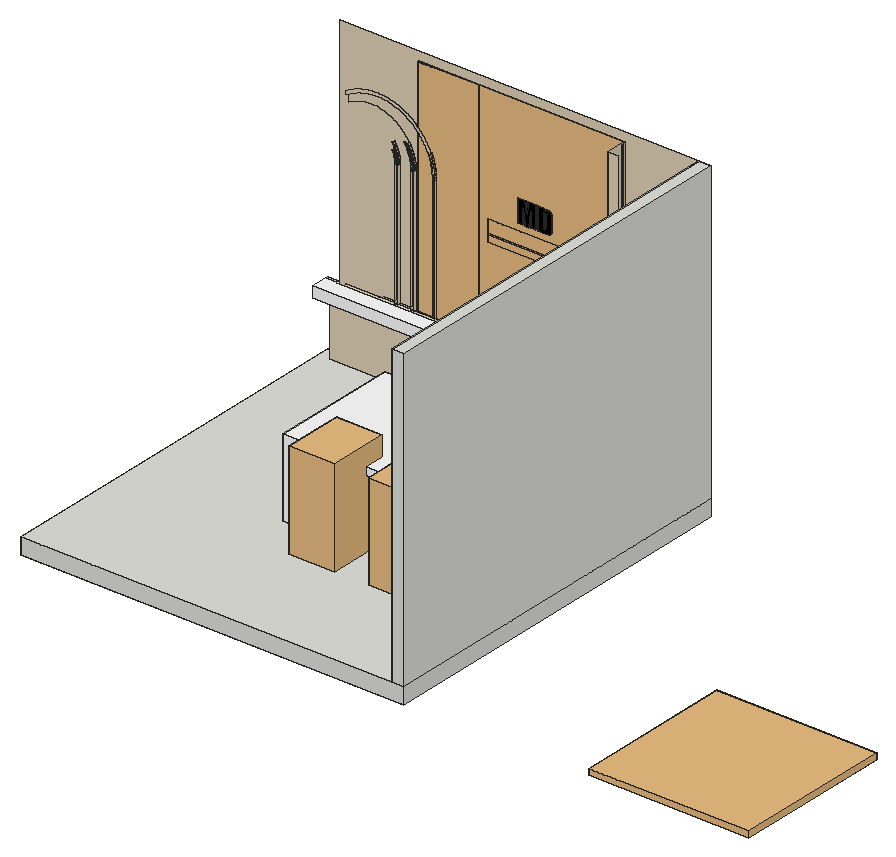
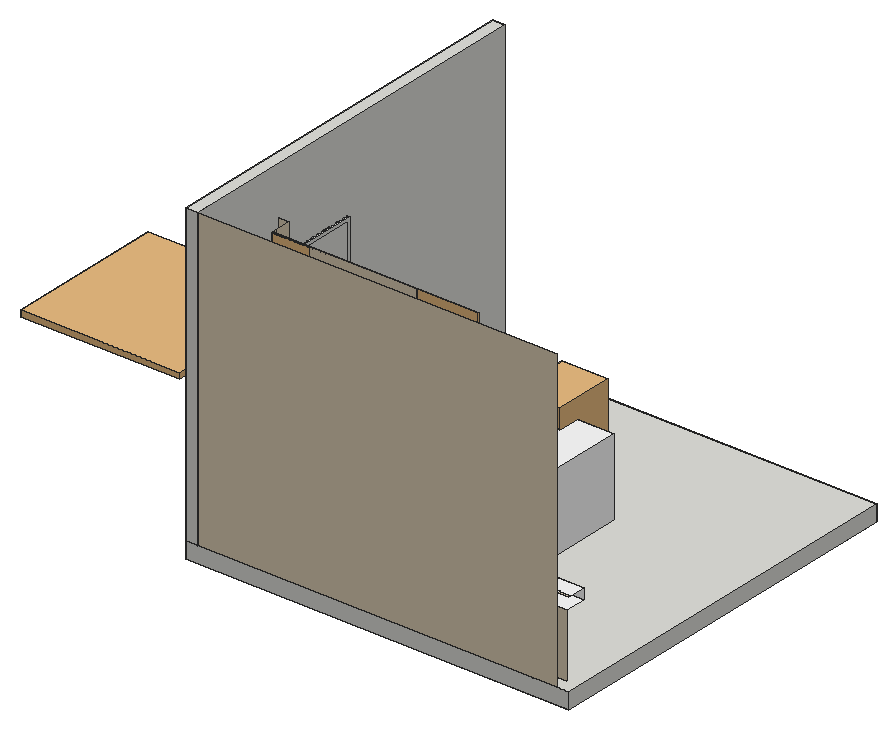
# SketchUp Ruby script. Lengths in inches.
U = 1.inch
M = Sketchup.active_model
def pt(a) = Geom::Point3d.new(a.map { |v| v * U })
def face(e, loops, mat)
  f = e.add_face(loops[0].map { |a| pt(a) })
  loops[1..].each { |l| e.add_face(l.map { |a| pt(a) }).erase! }
  f.material = f.back_material = mat if mat
  f
end
# faces: each face lists its corners as indices into pts; further lists are holes
def faces(e, pts, list, mat = nil) = list.each { |f| face(e, (f[0].is_a?(Array) ? f : [f]).map { |l| l.map { |i| pts[i] } }, mat) }
# xy, xz, yz: faces in a plane at the given z, y or x. An outline is a flat list of corners, or four numbers for a rectangle; further outlines are holes
def ring(l) = l.size == 4 ? [[l[0], l[1]], [l[2], l[1]], [l[2], l[3]], [l[0], l[3]]] : l.each_slice(2).to_a
def flat(e, list, mat, &to3) = list.each { |f| face(e, (f[0].is_a?(Array) ? f : [f]).map { |l| ring(l).map { |u, v| to3.(u, v) } }, mat) }
def xy(e, z, list, mat = nil) = flat(e, list, mat) { |x, y| [x, y, z] }
def xz(e, y, list, mat = nil) = flat(e, list, mat) { |x, z| [x, y, z] }
def yz(e, x, list, mat = nil) = flat(e, list, mat) { |y, z| [x, y, z] }
def lines(e, pts, list) = list.each { |a, b| e.add_line(pt(pts[a]), pt(pts[b])) }
# prism: a flat outline (further loops are holes) pulled along v
def prism(e, loops, v, mat = nil)
  f = face(e, loops, mat); d = Geom::Vector3d.new(v.map { |x| x * U })
  f.pushpull(f.normal.samedirection?(d) ? d.length : -d.length)
end
def box(e, o, s, mat = nil) = prism(e, [[o, [o[0] + s[0], o[1], o[2]], [o[0] + s[0], o[1] + s[1], o[2]], [o[0], o[1] + s[1], o[2]]]], [0, 0, s[2]], mat)
def at(x, y, z, deg = 0) = Geom::Transformation.translation(pt([x, y, z])) * Geom::Transformation.rotation(ORIGIN, Z_AXIS, deg.degrees)
def axes(o, x, y, z) = Geom::Transformation.new([*x, 0, *y, 0, *z, 0, *pt(o).to_a, 1])
def part(name) = M.definitions.add(name)
# library, detail: a bought-in or finely detailed component or shape, given as its bounding box
def library(name, o, s) = part(name).tap { |d| box(d.entities, o, s) }
def detail(e, o, s) = box(e.add_group.entities, o, s)
def put(e, d, t, mat = nil) = e.add_instance(d, t).tap { |i| i.material = mat if mat }
def group(e, t, mat = nil) = e.add_group.tap { |g| g.transformation = t; g.material = mat if mat }.entities
root = M.entities
M.materials.add("Oak Veneered MDF (Z8GPD2)").color = [209, 167, 120]
M.materials.add("Teddy_Brim").color = [225, 210, 185]
M.materials.add("[Color M00]").color = [255, 255, 255]
M.materials.add("[Color M09]").color = [0, 0, 0]
M.materials.add("[Color_000]").color = [255, 255, 255]
M.materials.add("[Color_D05]1").color = [255, 242, 204]
c1 = library("Group10\#1",[-11.375,-42,0],[22.75,84,0.5])
c2 = library("silla generica",[-12.64,0.67,0],[23.23,30.27,48.95])
c3 = part("MD")
prism(c3.entities,[[[3.42,4,0],[3.42,0,0],[2.51,0,0],[2.51,2.7,0],[2.14,0,0],[1.5,0,0],[1.12,2.64,0],[1.12,0,0],[0.21,0,0],[0.21,4,0],[1.55,4,0],[1.68,3.15,0],[1.82,2.13,0],[2.0625,4,0]]],[0,0,2])
prism(c3.entities,[[[3.83,4,0],[4.61,4,0],[5.24,3.98,0],[5.63,3.93,0],[5.87,3.84,0],[6.04,3.7,0],[6.15,3.54,0],[6.21,3.35,0],[6.24,2.59,0],[6.24,1.1875,0],[6.23,0.74,0],[6.19,0.47,0],[6.125,0.31,0],[6.02,0.18,0],[5.875,0.1,0],[5.7,0.04,0],[5.15,0,0],[3.83,0,0]],[[4.875,3.32,0],[4.875,0.68,0],[5.06,0.71,0],[5.15,0.77,0],[5.19,0.94,0],[5.2,1.26,0],[5.2,2.82,0],[5.1875,3.17,0],[5.11,3.28,0]]],[0,0,2])
c4 = library("Architexures|int",[-0.02,0,0],[30.58,2.32,2])
c5 = library("master design st",[0.17,0,0],[35.89,4.7,2])
c6 = library("Group34\#2",[-27.2,-42,0],[54.4,84,0.5])
c7 = library("chairs office (2)",[-15.11,-13.4,-0.04],[27.95,30.25,45.94])
c8 = library("laptop",[-0.05,16.1,0.9],[15.46,16.39,10.55])
c9 = library("Pen",[0.21,0.93,0.15],[2.77,2.76,4.45])
c10 = part("Closed book \#1")
xy(c10.entities,0,[[0.12,0.12,1.66,6.72]])
xy(c10.entities,0,[[0,0,0,6.8,0.12,6.8,0.12,0.12,1.66,0.12,1.66,6.8,1.77,6.8,1.77,0]],"[Color_000]")
xy(c10.entities,9.22,[[0.12,0.12,1.66,6.72]],"[Color_D05]1")
xy(c10.entities,9.33,[[0,0,1.77,0,1.77,6.8,1.66,6.8,1.66,0.12,0.12,0.12,0.12,6.8,0,6.8]],"[Color_000]")
xz(c10.entities,0,[[0,0,1.77,9.33]])
xz(c10.entities,0.12,[[0.12,0,1.66,9.22]])
xz(c10.entities,0.12,[[0.12,9.22,1.66,9.33]],"[Color_000]")
xz(c10.entities,6.72,[[0.12,0,1.66,9.22]],"[Color_D05]1")
xz(c10.entities,6.8,[[0,0,0.12,9.33],[1.66,0,1.77,9.33]],"[Color_000]")
yz(c10.entities,0,[[0,0,6.8,9.33]])
yz(c10.entities,0.12,[[0.12,0,6.72,9.22]])
yz(c10.entities,0.12,[[6.72,0,6.8,0,6.8,9.33,0.12,9.33,0.12,9.22,6.72,9.22]],"[Color_000]")
yz(c10.entities,1.66,[[0.12,0,6.72,9.22]])
yz(c10.entities,1.66,[[6.72,0,6.72,9.22,0.12,9.22,0.12,9.33,6.8,9.33,6.8,0]],"[Color_000]")
yz(c10.entities,1.77,[[0,0,6.8,9.33]])
c11 = part("Closed book \#2")
xy(c11.entities,0,[[0.12,0.12,1.11,7.59]])
xy(c11.entities,0,[[0,0,0,7.67,0.12,7.67,0.12,0.12,1.11,0.12,1.11,7.67,1.22,7.67,1.22,0]],"[Color_000]")
xy(c11.entities,10.875,[[0.12,0.12,1.11,7.59]],"[Color_D05]1")
xy(c11.entities,10.99,[[0,0,1.22,0,1.22,7.67,1.11,7.67,1.11,0.12,0.12,0.12,0.12,7.67,0,7.67]],"[Color_000]")
xz(c11.entities,0,[[0,0,1.22,10.99]])
xz(c11.entities,0.12,[[0.12,0,1.11,10.875]])
xz(c11.entities,0.12,[[0.12,10.875,1.11,10.99]],"[Color_000]")
xz(c11.entities,7.59,[[0.12,0,1.11,10.875]],"[Color_D05]1")
xz(c11.entities,7.67,[[0,0,0.12,10.99]])
xz(c11.entities,7.67,[[1.11,0,1.22,10.99]],"[Color_000]")
yz(c11.entities,0,[[0,0,7.67,10.99]])
yz(c11.entities,0.12,[[0.12,0,7.59,10.875]])
yz(c11.entities,0.12,[[7.59,0,7.67,0,7.67,10.99,0.12,10.99,0.12,10.875,7.59,10.875]],"[Color_000]")
yz(c11.entities,1.11,[[0.12,0,7.59,10.875]])
yz(c11.entities,1.11,[[7.59,0,7.59,10.875,0.12,10.875,0.12,10.99,7.67,10.99,7.67,0]],"[Color_000]")
yz(c11.entities,1.22,[[0,0,7.67,10.99]])
c12 = part("Closed book")
xy(c12.entities,0,[[0.12,0.12,0.99,5.93]])
xy(c12.entities,0,[[0,0,0,6.01,0.12,6.01,0.12,0.12,0.99,0.12,0.99,6.01,1.1,6.01,1.1,0]],"[Color_000]")
xy(c12.entities,9.5,[[0.12,0.12,0.99,5.93]],"[Color_D05]1")
xy(c12.entities,9.61,[[0,0,1.1,0,1.1,6.01,0.99,6.01,0.99,0.12,0.12,0.12,0.12,6.01,0,6.01]],"[Color_000]")
xz(c12.entities,0,[[0,0,1.1,4.45],[0,4.45,1.1,9.61]])
xz(c12.entities,0.12,[[0.12,0,0.99,9.5]])
xz(c12.entities,0.12,[[0.12,9.5,0.99,9.61]],"[Color_000]")
xz(c12.entities,5.93,[[0.12,0,0.99,9.5]],"[Color_D05]1")
xz(c12.entities,6.01,[[0,0,0.12,9.61],[0.99,0,1.1,9.61]],"[Color_000]")
yz(c12.entities,0,[[0,0,6.01,9.61]])
yz(c12.entities,0.12,[[0.12,0,5.93,9.5]])
yz(c12.entities,0.12,[[5.93,0,6.01,0,6.01,9.61,0.12,9.61,0.12,9.5,5.93,9.5]],"[Color_000]")
yz(c12.entities,0.99,[[0.12,0,5.93,9.5]])
yz(c12.entities,0.99,[[5.93,0,5.93,9.5,0.12,9.5,0.12,9.61,6.01,9.61,6.01,0]],"[Color_000]")
yz(c12.entities,1.1,[[0,0,6.01,9.61]])
c13 = part("Closed book \#3")
xy(c13.entities,0,[[0.12,0.12,0.68,7.875]])
xy(c13.entities,0,[[0,0,0,7.95,0.12,7.95,0.12,0.12,0.68,0.12,0.68,7.95,0.79,7.95,0.79,0]],"[Color_000]")
xy(c13.entities,9.5,[[0.12,0.12,0.68,7.875]],"[Color_D05]1")
xy(c13.entities,9.61,[[0,0,0.79,0,0.79,7.95,0.68,7.95,0.68,0.12,0.12,0.12,0.12,7.95,0,7.95]],"[Color_000]")
xz(c13.entities,0,[[0,0,0.79,9.61]])
xz(c13.entities,0.12,[[0.12,0,0.68,9.5]])
xz(c13.entities,0.12,[[0.12,9.5,0.68,9.61]],"[Color_000]")
xz(c13.entities,7.875,[[0.12,0,0.68,9.5]],"[Color_D05]1")
xz(c13.entities,7.95,[[0,0,0.12,9.61],[0.68,0,0.79,9.61]],"[Color_000]")
yz(c13.entities,0,[[0,0,7.95,9.61]])
yz(c13.entities,0.12,[[0.12,0,7.875,9.5]])
yz(c13.entities,0.12,[[7.875,0,7.95,0,7.95,9.61,0.12,9.61,0.12,9.5,7.875,9.5]],"[Color_000]")
yz(c13.entities,0.68,[[0.12,0,7.875,9.5]])
yz(c13.entities,0.68,[[7.875,0,7.875,9.5,0.12,9.5,0.12,9.61,7.95,9.61,7.95,0]],"[Color_000]")
yz(c13.entities,0.79,[[0,0,7.95,9.61]])
c14 = part("Stack of books")
put(c14.entities,c10,axes([0.4,0.3125,3],[0,0,-1],[0,1.5,0],[1.344,0,0]))
put(c14.entities,c11,axes([0,0,1.22],[0,0,-1],[0,1.5,0],[1.236,0,0]))
put(c14.entities,c12,axes([0.65,0.3125,4.1],[0,0,-1],[0,1.5,0],[1.2,0,0]))
put(c14.entities,c13,axes([1.65,0.75,4.89],[0,0,-1],[0,1,0],[1,0,0]))
c15 = library("Interior Props 221 030",[-2.57,-3.63,-0.04],[5.13,7.27,11.89])
c16 = library("Decorative Deer 97-30",[-7.23,-2.03,0],[14.46,4,11.8125])
c17 = library("Alarm Clock 114 007",[-2.86,-1.17,0.01],[5.71,2.99,7.86])
xy(root,6,[[4.5,139.5,139.5,144]],"Teddy_Brim")
xy(root,30,[[99.125,131.5,103.125,139.5]],"Teddy_Brim")
xy(root,30,[[4.5,131.5,99.125,139.5]],"[Color M00]")
xy(root,30.14,[[105.21,131.5,139.5,139.5]],"Teddy_Brim")
xy(root,34,[[113.66,131.5,139.5,139.5],[23.86,138.5,23.86,138.6875,99.125,138.6875,99.125,139.5,44.86,139.5,44.86,138.5,43.86,138.5,43.86,139.5,36.86,139.5,36.86,138.5,35.86,138.5,35.86,139.5,30.86,139.5,30.86,138.5,29.86,138.5,29.86,139.5,24.86,139.5,24.86,138.5],[29.86,138.5,30.86,138.6875],[35.86,138.5,36.86,138.6875],[43.86,138.5,44.86,138.6875]],"Teddy_Brim")
xy(root,34,[[4.5,131.5,99.125,131.5,99.125,137.6875,11.5,137.6875,11.5,137.5,8.5,137.5,8.5,137.6875,4.5,137.6875]],"[Color M00]")
xy(root,46,[[119.125,131.5,139.5,139.5]],"Teddy_Brim")
xy(root,46.79,[[119.125,131.5,139.5,139.5]],"Teddy_Brim")
xy(root,69.61,[[119.125,131.5,139.5,138.79]],"Teddy_Brim")
xy(root,70.39,[[119.125,131.5,139.5,139.5]],"Teddy_Brim")
xz(root,131.5,[[99.125,30,103.125,30,105.21,30.14,107.27,30.55,109.25,31.22,111.125,32.14,112.87,33.31,113.66,34,114.4375,34.6875,115.125,35.47,115.82,36.26,116.98,38,117.91,39.88,118.58,41.86,118.99,43.91,119.125,46,119.125,118,115.125,118,115.125,52,115.23,49.74,115.125,48.6,115.02,47.48,114.49,45.28,113.67,43.17,112.55,41.2,111.17,39.41,109.55,37.82,107.72,36.48,105.73,35.41,103.6,34.63,101.38,34.16,99.125,34],[105.21,30.14,139.5,30.14,139.5,34,113.66,34,112.87,33.31,111.125,32.14,109.25,31.22,107.27,30.55],[119.125,46,139.5,46.79],[119.125,69.61,139.5,70.39]],"Teddy_Brim")
xz(root,131.5,[[4.5,30,99.125,34]],"[Color M00]")
xz(root,138.5,[[43.86,34,44.86,34,44.86,80.61,44.85,81.08,44.84,81.54,44.8125,82,44.78,82.47,44.68,83.39,44.62,83.85,44.54,84.31,44.46,84.76,44.37,85.22,44.15,86.12,44.03,86.57,43.89,87.01,43.75,87.46,43.6,87.89,43.44,88.33,43.1,89.19,42.91,89.62,42.71,90.04,42.51,90.45,42.07,91.27,41.84,91.67,41.6,92.07,41.35,92.46,41.09,92.85,40.82,93.23,40.55,93.6,40.27,93.97,39.98,94.34,39.38,95.04,39.07,95.39,38.75,95.72,38.09,96.38,37.75,96.69,37.4,97,37.05,97.3,36.69,97.6,36.33,97.88,35.96,98.16,35.58,98.43,35.19,98.69,34.81,98.95,34.72,99,34.41,99.19,34.01,99.43,33.61,99.66,33.2,99.88,32.79,100.09,32.37,100.29,31.95,100.48,31.52,100.67,30.66,101.01,30.22,101.16,29.78,101.3125,29.34,101.45,28.89,101.58,28.44,101.7,27.54,101.9,27.08,101.99,26.625,102.07,26.17,102.14,25.71,102.2,25.25,102.25,24.78,102.3,24.32,102.33,23.86,102.35,23.39,102.36,22.93,102.36,22.46,102.35,22,102.33,21.54,102.3,21.08,102.26,20.61,102.22,20.15,102.16,19.69,102.09,19.24,102.01,18.78,101.92,18.33,101.83,17.875,101.72,17.43,101.6,16.98,101.48,16.1,101.2,15.22,100.88,14.79,100.71,14.37,100.52,13.94,100.33,13.52,100.13,12.7,99.71,12.3,99.48,11.5,99,11.5,97.85,12.5,98.4375,12.79,98.61,13.18,98.83,13.57,99.04,13.97,99.23,14.36,99.43,14.77,99.61,15.59,99.95,16,100.1,16.42,100.25,16.84,100.39,17.26,100.52,17.6875,100.64,18.12,100.75,18.55,100.85,18.98,100.94,19.42,101.03,19.85,101.1,20.29,101.17,21.17,101.27,21.61,101.31,22.49,101.35,22.9375,101.36,23.38,101.36,23.82,101.35,24.26,101.33,24.71,101.3,25.15,101.26,25.59,101.21,26.03,101.15,26.46,101.09,26.9,101.01,27.33,100.93,27.77,100.83,28.2,100.73,29.05,100.49,29.47,100.36,29.89,100.22,30.3125,100.07,30.72,99.91,31.13,99.75,31.54,99.57,31.94,99.39,32.74,98.99,33.125,98.78,33.51,98.5625,33.89,98.34,34.19,98.15,34.27,98.1,34.64,97.86,35,97.61,35.72,97.09,36.07,96.82,36.41,96.54,36.75,96.25,37.08,95.95,37.4,95.65,37.72,95.34,38.03,95.03,38.34,94.71,38.92,94.05,39.21,93.7,39.48,93.36,39.75,93.01,40.01,92.65,40.26,92.29,40.51,91.92,40.75,91.54,40.98,91.16,41.2,90.78,41.41,90.39,41.61,90,41.81,89.6,42,89.2,42.18,88.8,42.35,88.39,42.51,87.98,42.66,87.56,42.8,87.14,42.9375,86.72,43.07,86.3,43.18,85.87,43.29,85.4375,43.39,85.01,43.48,84.57,43.56,84.14,43.63,83.7,43.6875,83.26,43.74,82.82,43.82,81.94,43.84,81.5,43.85,81.06,43.86,80.61]],"Teddy_Brim")
xz(root,139.5,[[4.5,6,139.5,6,139.5,30.14,105.21,30.14,103.125,30,4.5,30],[36.86,34,43.86,34,43.86,80.61,43.85,81.06,43.84,81.5,43.82,81.94,43.74,82.82,43.6875,83.26,43.63,83.7,43.56,84.14,43.48,84.57,43.39,85.01,43.29,85.4375,43.18,85.87,43.07,86.3,42.9375,86.72,42.8,87.14,42.66,87.56,42.51,87.98,42.35,88.39,42.18,88.8,42,89.2,41.81,89.6,41.61,90,41.41,90.39,41.2,90.78,40.98,91.16,40.75,91.54,40.51,91.92,40.26,92.29,40.01,92.65,39.75,93.01,39.48,93.36,39.21,93.7,38.92,94.05,38.34,94.71,38.03,95.03,37.72,95.34,37.4,95.65,37.08,95.95,36.75,96.25,36.41,96.54,36.07,96.82,35.72,97.09,35,97.61,34.64,97.86,34.27,98.1,34.19,98.15,33.89,98.34,33.51,98.5625,33.125,98.78,32.74,98.99,31.94,99.39,31.54,99.57,31.13,99.75,30.72,99.91,30.3125,100.07,29.89,100.22,29.47,100.36,29.05,100.49,28.2,100.73,27.77,100.83,27.33,100.93,26.9,101.01,26.46,101.09,26.03,101.15,25.59,101.21,25.15,101.26,24.71,101.3,24.26,101.33,23.82,101.35,23.38,101.36,22.9375,101.36,22.49,101.35,21.61,101.31,21.17,101.27,20.29,101.17,19.85,101.1,19.42,101.03,18.98,100.94,18.55,100.85,18.12,100.75,17.6875,100.64,17.26,100.52,16.84,100.39,16.42,100.25,16,100.1,15.59,99.95,14.77,99.61,14.36,99.43,13.97,99.23,13.57,99.04,13.18,98.83,12.79,98.61,12.5,98.4375,11.5,97.85,11.5,95,11.81,95.18,12.11,95.35,12.43,95.52,12.74,95.67,13.0625,95.83,13.38,95.97,13.71,96.11,14.37,96.37,14.7,96.48,15.04,96.6,15.72,96.8,16.06,96.88,16.4,96.97,17.1,97.11,17.45,97.17,18.15,97.27,19.2,97.36,19.56,97.37,19.91,97.38,20.26,97.38,20.62,97.375,20.97,97.36,21.32,97.34,21.68,97.31,22.38,97.23,22.73,97.17,23.08,97.12,23.42,97.05,23.77,96.98,24.11,96.89,24.46,96.81,25.14,96.61,25.47,96.5,25.81,96.38,26.14,96.26,26.47,96.13,26.79,95.99,27.12,95.84,27.43,95.69,27.75,95.54,28.375,95.2,28.68,95.02,28.98,94.84,29.28,94.65,29.86,94.25,30.15,94.04,30.71,93.6,30.98,93.375,31.24,93.14,31.51,92.91,32.26,92.16,32.74,91.64,32.96,91.37,33.1875,91.09,33.41,90.81,33.62,90.53,34.22,89.66,34.41,89.36,34.59,89.05,34.76,88.75,34.93,88.43,35.09,88.12,35.25,87.8,35.39,87.48,35.54,87.16,35.8,86.5,35.92,86.17,36.14,85.49,36.24,85.15,36.33,84.8125,36.41,84.47,36.49,84.125,36.56,83.78,36.68,83.08,36.73,82.73,36.77,82.38,36.8,82.03,36.83,81.67,36.85,80.97,36.86,80.61],[113.66,34,139.5,34,139.5,46,119.125,46,118.99,43.91,118.58,41.86,117.91,39.88,116.98,38,115.82,36.26,115.125,35.47,114.4375,34.6875],[60.73,46,97.125,46,97.65,46.03,98.16,46.14,98.66,46.3,99.125,46.54,99.56,46.83,99.95,47.17,100.3,47.56,100.59,48,100.82,48.47,100.99,48.96,101.09,49.48,101.125,50,101.125,118,60.73,118],[119.125,46.79,139.5,69.61],
  [115.125,48.6,115.23,49.74,115.125,52],[119.125,70.39,139.5,93.61]],"Teddy_Brim")
xz(root,144,[[4.5,6,139.5,118]],"Teddy_Brim")
yz(root,29.86,[[138.5,34,139.5,35],[138.5,35,139,80.62]],"Teddy_Brim")
yz(root,30.86,[[138.5,34,139.5,80.61],[138.5,80.61,139.5,80.88],[138.5,80.88,139.5,81.15]],"Teddy_Brim")
yz(root,35.86,[[138.5,34,139.5,35],[138.5,35,139,80.61],[138.5,80.61,139,80.95]],"Teddy_Brim")
yz(root,36.86,[[138.5,34,139.5,80.61]],"Teddy_Brim")
yz(root,43.86,[[138.5,34,139.5,35],[138.5,35,139,80.61]],"Teddy_Brim")
yz(root,44.86,[[138.5,34,139.5,80.61]],"Teddy_Brim")
yz(root,115.125,[[131.5,52,137.6875,118],[138.6875,52,139.5,118]],"Teddy_Brim")
yz(root,119.125,[[131.5,46.79,139.5,69.61],[131.5,70.39,139.5,93.61]],"Teddy_Brim")
yz(root,139.5,[[139.5,6,144,6,144,118,139.5,118,139.5,94.39,131.5,94.39,131.5,93.61,139.5,93.61,139.5,70.39,131.5,70.39,131.5,69.61,139.5,69.61,139.5,46.79,131.5,46.79,131.5,46,139.5,46,139.5,34,131.5,34,131.5,30.14,139.5,30.14]],"Teddy_Brim")
p = [[103.125,139.5,30],[105.21,139.5,30.14],[105.21,131.5,30.14],[103.125,131.5,30],[101.38,131.5,34.16],[101.38,137.6875,34.16],
  [99.125,137.6875,34],[99.125,131.5,34],[113.66,139.5,34],[114.4375,139.5,34.6875],[114.4375,131.5,34.6875],[113.66,131.5,34],
  [99.125,139.5,34],[99.125,138.6875,34],[101.38,138.6875,34.16],[101.38,139.5,34.16],[103.6,131.5,34.63],[103.6,137.6875,34.63],
  [103.6,138.6875,34.63],[103.6,139.5,34.63],[105.73,131.5,35.41],[105.73,137.6875,35.41],[105.73,138.6875,35.41],[105.73,139.5,35.41],
  [115.125,139.5,35.47],[115.125,131.5,35.47],[107.72,131.5,36.48],[107.72,137.6875,36.48],[107.72,138.6875,36.48],[107.72,139.5,36.48],
  [115.82,139.5,36.26],[115.82,131.5,36.26],[116.98,139.5,38],[116.98,131.5,38],[109.55,131.5,37.82],[109.55,137.6875,37.82],
  [109.55,138.6875,37.82],[109.55,139.5,37.82],[111.17,131.5,39.41],[111.17,137.6875,39.41],[111.17,138.6875,39.41],[111.17,139.5,39.41],
  [117.91,139.5,39.88],[117.91,131.5,39.88],[112.55,131.5,41.2],[112.55,137.6875,41.2],[112.55,138.6875,41.2],[112.55,139.5,41.2],
  [118.58,139.5,41.86],[118.58,131.5,41.86],[113.67,131.5,43.17],[113.67,137.6875,43.17],[113.67,138.6875,43.17],[113.67,139.5,43.17],
  [118.99,139.5,43.91],[118.99,131.5,43.91],[114.49,131.5,45.28],[114.49,137.6875,45.28],[114.49,138.6875,45.28],[114.49,139.5,45.28],
  [119.125,139.5,46],[119.125,131.5,46],[115.02,131.5,47.48],[115.02,137.6875,47.48],[115.02,138.6875,47.48],[115.02,139.5,47.48],
  [115.125,131.5,48.6],[115.125,137.6875,48.6],[115.125,138.6875,48.6],[115.125,139.5,48.6],[115.23,131.5,49.74],[115.23,137.6875,49.74],
  [115.23,138.6875,49.74],[115.23,139.5,49.74],[115.125,131.5,52],[115.125,137.6875,52],[115.125,138.6875,52],[115.125,139.5,52],
  [29.85,138.5,80.89],[29.85,139,80.89],[29.86,139,80.62],[29.86,138.5,80.62],[36.86,139.5,80.61],[36.85,139.5,80.97],
  [36.85,138.5,80.97],[36.86,138.5,80.61],[43.85,138.5,81.06],[43.85,139,81.06],[43.86,139,80.61],[43.86,138.5,80.61],
  [44.86,139.5,80.61],[44.85,139.5,81.08],[44.85,138.5,81.08],[44.86,138.5,80.61],[29.84,138.5,81.15],[29.84,139,81.15],
  [35.84,138.5,81.28],[35.84,139,81.28],[35.86,139,80.95],[35.86,138.5,80.95],[36.84,139.5,81.32],[36.84,138.5,81.32],
  [29.82,138.5,81.4],[29.82,139,81.4],[43.84,138.5,81.5],[43.84,139,81.5],[44.84,139.5,81.54],[44.84,138.5,81.54],
  [30.86,139.5,81.15],[30.85,139.5,81.43],[30.85,138.5,81.43],[30.86,138.5,81.15],[35.83,138.5,81.61],[35.83,139,81.61],
  [36.83,139.5,81.67],[36.83,138.5,81.67],[29.79,138.5,81.66],[29.79,139,81.66],[30.83,139.5,81.7],[30.83,138.5,81.7],
  [43.82,138.5,81.94],[43.82,139,81.94],[44.8125,139.5,82],[44.8125,138.5,82],[35.8,138.5,81.94],[35.8,139,81.94],
  [29.76,138.5,81.92],[29.76,139,81.92],[30.81,139.5,81.97],[30.81,138.5,81.97],[36.8,139.5,82.03],[36.8,138.5,82.03],
  [29.72,138.5,82.17],[29.72,139,82.17],[35.77,138.5,82.27],[35.77,139,82.27],[43.78,138.5,82.38],[43.78,139,82.38],
  [30.78,139.5,82.24],[30.78,138.5,82.24],[36.77,139.5,82.38],[36.77,138.5,82.38],[44.78,139.5,82.47],[44.78,138.5,82.47],
  [29.68,138.5,82.43],[29.68,139,82.43],[30.75,139.5,82.5],[30.75,138.5,82.5],[35.73,138.5,82.6],[35.73,139,82.6],
  [29.63,138.5,82.68],[29.63,139,82.68],[36.73,139.5,82.73],[36.73,138.5,82.73],[43.74,138.5,82.82],[43.74,139,82.82],
  [30.71,139.5,82.77],[30.71,138.5,82.77],[44.73,139.5,82.93],[44.73,138.5,82.93],[35.6875,138.5,82.93],[35.6875,139,82.93],
  [29.58,138.5,82.93],[29.58,139,82.93],[36.68,139.5,83.08],[36.68,138.5,83.08],[30.67,139.5,83.04],[30.67,138.5,83.04],
  [43.6875,138.5,83.26],[43.6875,139,83.26],[29.52,138.5,83.18],[29.52,139,83.18],[35.64,138.5,83.26],[35.64,139,83.26],
  [44.68,139.5,83.39],[44.68,138.5,83.39],[30.61,139.5,83.31],[30.61,138.5,83.31],[36.62,139.5,83.43],[36.62,138.5,83.43],
  [29.46,138.5,83.43],[29.46,139,83.43],[30.56,139.5,83.57],[30.56,138.5,83.57],[35.58,138.5,83.59],[35.58,139,83.59],
  [43.63,138.5,83.7],[43.63,139,83.7],[29.39,138.5,83.68],[29.39,139,83.68],[36.56,139.5,83.78],[36.56,138.5,83.78],
  [44.62,139.5,83.85],[44.62,138.5,83.85],[30.5,139.5,83.83],[30.5,138.5,83.83],[35.51,138.5,83.92],[35.51,139,83.92],
  [29.3125,138.5,83.92],[29.3125,139,83.92],[43.56,138.5,84.14],[43.56,139,84.14],[30.43,139.5,84.1],[30.43,138.5,84.1],
  [36.49,139.5,84.125],[36.49,138.5,84.125],[44.54,139.5,84.31],[44.54,138.5,84.31],[29.23,138.5,84.17],[29.23,139,84.17],
  [35.4375,138.5,84.24],[35.4375,139,84.24],[30.35,139.5,84.36],[30.35,138.5,84.36],[36.41,139.5,84.47],[36.41,138.5,84.47],
  [43.48,138.5,84.57],[43.48,139,84.57],[29.15,138.5,84.41],[29.15,139,84.41],[35.36,138.5,84.5625],[35.36,139,84.5625],
  [44.46,139.5,84.76],[44.46,138.5,84.76],[29.05,138.5,84.65],[29.05,139,84.65],[30.27,139.5,84.62],[30.27,138.5,84.62],
  [36.33,139.5,84.8125],[36.33,138.5,84.8125],[30.1875,139.5,84.87],[30.1875,138.5,84.87],[35.27,138.5,84.88],[35.27,139,84.88],
  [43.39,138.5,85.01],[43.39,139,85.01],[28.96,138.5,84.89],[28.96,139,84.89],[36.24,139.5,85.15],[36.24,138.5,85.15],
  [44.37,139.5,85.22],[44.37,138.5,85.22],[28.86,138.5,85.13],[28.86,139,85.13],[30.1,139.5,85.13],[30.1,138.5,85.13],
  [35.18,138.5,85.2],[35.18,139,85.2],[43.29,138.5,85.4375],[43.29,139,85.4375],[28.75,138.5,85.36],[28.75,139,85.36],
  [30,139.5,85.38],[30,138.5,85.38],[35.08,138.5,85.52],[35.08,139,85.52],[36.14,139.5,85.49],[36.14,138.5,85.49],
  [44.26,139.5,85.67],[44.26,138.5,85.67],[29.9,139.5,85.63],[29.9,138.5,85.63],[43.18,138.5,85.87],[43.18,139,85.87],
  [34.97,138.5,85.84],[34.97,139,85.84],[36.03,139.5,85.83],[36.03,138.5,85.83],[29.79,139.5,85.88],[29.79,138.5,85.88],
  [44.15,139.5,86.12],[44.15,138.5,86.12],[34.86,138.5,86.15],[34.86,139,86.15],[35.92,139.5,86.17],[35.92,138.5,86.17],
  [29.68,139.5,86.125],[29.68,138.5,86.125],[43.07,138.5,86.3],[43.07,139,86.3],[29.56,139.5,86.37],[29.56,138.5,86.37],
  [34.74,138.5,86.46],[34.74,139,86.46],[44.03,139.5,86.57],[44.03,138.5,86.57],[35.8,139.5,86.5],[35.8,138.5,86.5],
  [42.9375,138.5,86.72],[42.9375,139,86.72],[29.43,139.5,86.61],[29.43,138.5,86.61],[34.61,138.5,86.77],[34.61,139,86.77],
  [35.67,139.5,86.83],[35.67,138.5,86.83],[29.31,139.5,86.85],[29.31,138.5,86.85],[43.89,139.5,87.01],[43.89,138.5,87.01],
  [42.8,138.5,87.14],[42.8,139,87.14],[29.17,139.5,87.09],[29.17,138.5,87.09],[34.48,138.5,87.07],[34.48,139,87.07],
  [35.54,139.5,87.16],[35.54,138.5,87.16],[43.75,139.5,87.46],[43.75,138.5,87.46],[29.03,139.5,87.32],[29.03,138.5,87.32],
  [34.34,138.5,87.375],[34.34,139,87.375],[42.66,138.5,87.56],[42.66,139,87.56],[35.39,139.5,87.48],[35.39,138.5,87.48],
  [28.89,139.5,87.55],[28.89,138.5,87.55],[34.2,138.5,87.67],[34.2,139,87.67],[28.74,139.5,87.77],[28.74,138.5,87.77],
  [35.25,139.5,87.8],[35.25,138.5,87.8],[43.6,139.5,87.89],[43.6,138.5,87.89],[42.51,138.5,87.98],[42.51,139,87.98],
  [34.04,138.5,87.97],[34.04,139,87.97],[35.09,139.5,88.12],[35.09,138.5,88.12],[43.44,139.5,88.33],[43.44,138.5,88.33],
  [33.89,138.5,88.26],[33.89,139,88.26],[42.35,138.5,88.39],[42.35,139,88.39],[34.93,139.5,88.43],[34.93,138.5,88.43],
  [33.72,138.5,88.55],[33.72,139,88.55],[43.27,139.5,88.76],[43.27,138.5,88.76],[34.76,139.5,88.75],[34.76,138.5,88.75],
  [42.18,138.5,88.8],[42.18,139,88.8],[33.55,138.5,88.84],[33.55,139,88.84],[34.59,139.5,89.05],[34.59,138.5,89.05],
  [33.375,138.5,89.12],[33.375,139,89.12],[42,138.5,89.2],[42,139,89.2],[43.1,139.5,89.19],[43.1,138.5,89.19],
  [33.19,138.5,89.4],[33.19,139,89.4],[34.41,139.5,89.36],[34.41,138.5,89.36],[60.73,139.5,34],[60.73,139.5,46]]
faces(root,p,[[0,1,2,3],[4,5,6,7],[8,9,10,11],[12,13,14,15],[16,17,5,4],[15,14,18,19],[20,21,17,16],[19,18,22,23],
  [9,24,25,10],[26,27,21,20],[23,22,28,29],[24,30,31,25],[30,32,33,31],[34,35,27,26],[29,28,36,37],[38,39,35,34],
  [37,36,40,41],[32,42,43,33],[44,45,39,38],[41,40,46,47],[42,48,49,43],[50,51,45,44],[47,46,52,53],[48,54,55,49],
  [56,57,51,50],[53,52,58,59],[54,60,61,55],[62,63,57,56],[59,58,64,65],[66,67,63,62],[65,64,68,69],[70,71,67,66],
  [69,68,72,73],[74,75,71,70],[73,72,76,77],[78,79,80,81],[82,83,84,85],[86,87,88,89],[90,91,92,93],[94,95,79,78],
  [96,97,98,99],[83,100,101,84],[102,103,95,94],[104,105,87,86],[91,106,107,92],[108,109,110,111],[112,113,97,96],[100,114,115,101],
  [116,117,103,102],[109,118,119,110],[120,121,105,104],[106,122,123,107],[124,125,113,112],[126,127,117,116],[118,128,129,119],[114,130,131,115],
  [132,133,127,126],[134,135,125,124],[136,137,121,120],[128,138,139,129],[130,140,141,131],[122,142,143,123],[144,145,133,132],[138,146,147,139],
  [148,149,135,134],[150,151,145,144],[140,152,153,141],[154,155,137,136],[146,156,157,147],[142,158,159,143],[160,161,149,148],[162,163,151,150],
  [152,164,165,153],[156,166,167,157],[168,169,155,154],[170,171,163,162],[172,173,161,160],[158,174,175,159],[166,176,177,167],[164,178,179,165],
  [180,181,171,170],[176,182,183,177],[184,185,173,172],[186,187,169,168],[188,189,181,180],[178,190,191,179],[174,192,193,175],[182,194,195,183],
  [196,197,185,184],[198,199,189,188],[200,201,187,186],[194,202,203,195],[190,204,205,191],[192,206,207,193],[208,209,199,198],[210,211,197,196],
  [202,212,213,203],[204,214,215,205],[216,217,201,200],[218,219,209,208],[220,221,211,210],[206,222,223,207],[224,225,219,218],[212,226,227,213],
  [214,228,229,215],[226,230,231,227],[232,233,221,220],[234,235,217,216],[236,237,225,224],[228,238,239,229],[222,240,241,223],[242,243,237,236],
  [230,244,245,231],[246,247,233,232],[248,249,235,234],[250,251,243,242],[244,252,253,245],[254,255,247,246],[238,256,257,239],[240,258,259,241],
  [252,260,261,253],[262,263,249,248],[264,265,255,254],[256,266,267,257],[260,268,269,261],[258,270,271,259],[272,273,265,264],[266,274,275,267],
  [268,276,277,269],[278,279,263,262],[276,280,281,277],[282,283,273,272],[270,284,285,271],[274,286,287,275],[288,289,279,278],[280,290,291,281],
  [292,293,283,282],[286,294,295,287],[290,296,297,291],[284,298,299,285],[300,301,289,288],[296,302,303,297],[304,305,293,292],[294,306,307,295],
  [298,308,309,299],[302,310,311,303],[312,313,305,304],[314,315,301,300],[306,316,317,307],[310,318,319,311],[320,321,313,312],[318,322,323,319],
  [316,324,325,317],[308,326,327,309],[328,329,315,314],[330,331,321,320],[324,332,333,325],[326,334,335,327],[336,337,331,330],[338,339,329,328],
  [332,340,341,333],[342,343,337,336],[334,344,345,335],[340,346,347,341],[348,349,339,338],[350,351,343,342],[346,352,353,347],[354,355,351,350],
  [356,357,349,348],[344,358,359,345],[360,361,355,354],[352,362,363,353]],"Teddy_Brim")
lines(root,p,[[364,365]])
detail(root,[212.42,0.93,0],[60,60,2.25])
put(root,c1,axes([49.36,139.5,76],[1,0,0],[0,0,1],[0,-1,0]),"Teddy_Brim")
g1 = group(root,at(4.5,137.6875,34),"Teddy_Brim")
xy(g1,0,[[0,0,4,1],[7,0,94.625,0,94.625,1,40.36,1,40.36,0.8125,39.36,0.8125,39.36,1,32.36,1,32.36,0.8125,31.36,0.8125,31.36,1,26.36,1,26.36,0.8125,25.36,0.8125,25.36,1,20.36,1,20.36,0.8125,7,0.8125]])
yz(g1,110.625,[[0,18,1,84]])
p = [[94.625,1,0],[94.625,0,0],[96.88,0,0.16],[96.88,1,0.16],[99.1,0,0.63],[99.1,1,0.63],
  [101.23,0,1.41],[101.23,1,1.41],[103.22,0,2.48],[103.22,1,2.48],[105.05,0,3.82],[105.05,1,3.82],
  [106.67,0,5.41],[106.67,1,5.41],[108.05,0,7.2],[108.05,1,7.2],[109.17,0,9.17],[109.17,1,9.17],
  [109.99,0,11.28],[109.99,1,11.28],[110.52,0,13.48],[110.52,1,13.48],[110.625,0,14.6],[110.625,1,14.6],
  [110.73,0,15.74],[110.73,1,15.74],[110.625,0,18],[110.625,1,18]]
faces(g1,p,[[0,1,2,3],[3,2,4,5],[5,4,6,7],[7,6,8,9],[9,8,10,11],[11,10,12,13],[13,12,14,15],[15,14,16,17],
  [17,16,18,19],[19,18,20,21],[21,20,22,23],[23,22,24,25],[25,24,26,27]])
g2 = group(root,at(0,0,0))
box(g2,[0,0,0],[144,144,6])
put(root,c2,axes([77.21,63.88,6],[0.74,0,0],[0,-0.74,0],[0,0,0.74]))
put(root,c3,axes([75.12,139.5,76.86],[2.1,0,0],[0,0,2.1],[0,-0.315,0]),"[Color M09]")
put(root,c4,axes([64.22,139.5,66.68],[1.1628,0,0],[0,0,1],[0,-0.29,0]),"[Color M09]")
put(root,c5,axes([63.92,139.5,69.73],[1,0,0],[0,0,1],[0,-0.29,0]),"[Color M09]")
put(root,c6,axes([87.93,139.5,76],[1,0,0],[0,0,1],[0,-1,0]),"Teddy_Brim")
put(root,c7,at(89.32,107.03,6))
put(root,c8,at(113.8125,81.77,34.1,90))
g3 = group(root,at(54,55.5,6))
xy(g3,0,[[0,0,0,48,3,48,3,31,69,31,69,48,72,48,72,0,69,0,69,12,3,12,3,0]])
xy(g3,26,[[3,0,69,12],[3,31,69,48]])
xy(g3,29,[[0,0,72,48]],"[Color M00]")
xz(g3,0,[[0,0,3,0,3,26,69,26,69,0,72,0,72,29,0,29]],"[Color M00]")
xz(g3,12,[[3,0,69,26]],"Oak Veneered MDF (Z8GPD2)")
xz(g3,31,[[3,0,69,26]],"Oak Veneered MDF (Z8GPD2)")
xz(g3,48,[[0,0,0,29,72,29,72,0,69,0,69,26,3,26,3,0]],"[Color M00]")
yz(g3,0,[[0,0,48,29]],"[Color M00]")
yz(g3,3,[[0,0,12,26],[31,0,48,26]])
yz(g3,69,[[0,0,12,26]])
yz(g3,69,[[31,0,48,26]],"[Color M00]")
yz(g3,72,[[0,0,48,29]],"[Color M00]")
put(root,c9,at(102.22,87.03,34.85))
put(root,c2,axes([107.15,63.88,6],[0.74,0,0],[0,-0.74,0],[0,0,0.74]))
put(root,c14,at(106.59,86.94,35))
put(root,c15,at(126.53,135.68,46.79,-11.4))
put(root,c16,at(128.53,134.9375,70.39))
g4 = group(root,at(119.125,138.79,69.61),"Teddy_Brim")
xy(g4,0,[[0,0,20.375,0.71]])
put(root,c17,at(134.76,134.64,46.79))
g5 = group(root,at(138.52,73.75,50.09))
xy(g5,0,[[0,0,0.98,36]])
xy(g5,0.79,[[0,0.79,0.3125,35.21]])
xy(g5,35.21,[[0,0.79,0.3125,35.21]])
xy(g5,36,[[0,0,0.98,36]])
xz(g5,0,[[0,0,0.98,36]])
xz(g5,0.79,[[0,0.79,0.3125,35.21]])
xz(g5,35.21,[[0,0.79,0.3125,35.21]])
xz(g5,36,[[0,0,0.98,36]])
yz(g5,0,[[[0,0,36,36],[0.79,0.79,35.21,35.21]]])
yz(g5,0.3125,[[0.79,0.79,35.21,35.21]])
yz(g5,0.98,[[0,0,36,36]])
g6 = group(root,at(139.5,0,6))
box(g6,[0,0,0],[4.5,144,112])
